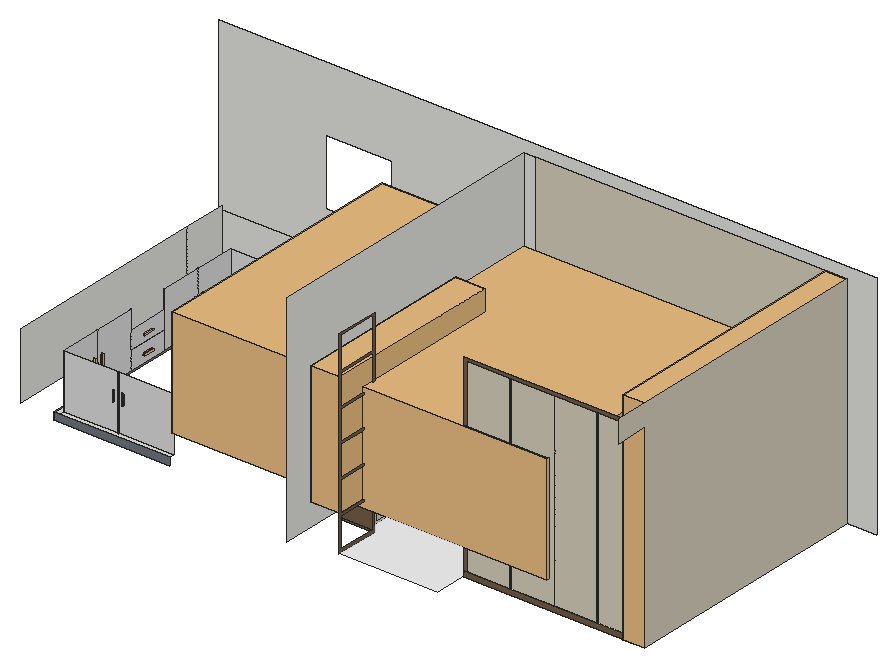
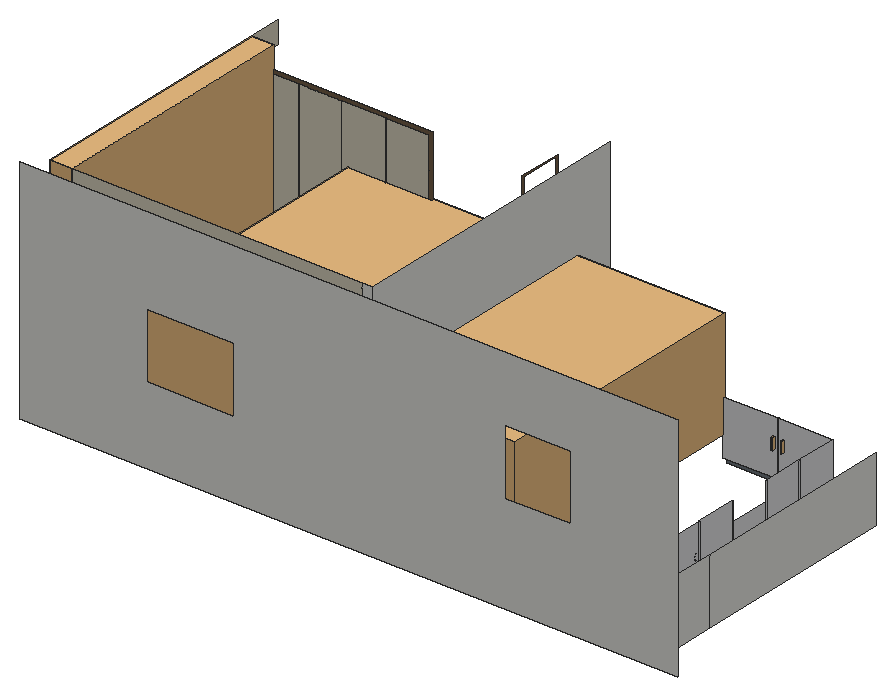
# SketchUp Ruby script. Lengths in inches.
U = 1.inch
M = Sketchup.active_model
def pt(a) = Geom::Point3d.new(a.map { |v| v * U })
def face(e, loops, mat)
  f = e.add_face(loops[0].map { |a| pt(a) })
  loops[1..].each { |l| e.add_face(l.map { |a| pt(a) }).erase! }
  f.material = f.back_material = mat if mat
  f
end
# faces: each face lists its corners as indices into pts; further lists are holes
def faces(e, pts, list, mat = nil) = list.each { |f| face(e, (f[0].is_a?(Array) ? f : [f]).map { |l| l.map { |i| pts[i] } }, mat) }
# xy, xz, yz: faces in a plane at the given z, y or x. An outline is a flat list of corners, or four numbers for a rectangle; further outlines are holes
def ring(l) = l.size == 4 ? [[l[0], l[1]], [l[2], l[1]], [l[2], l[3]], [l[0], l[3]]] : l.each_slice(2).to_a
def flat(e, list, mat, &to3) = list.each { |f| face(e, (f[0].is_a?(Array) ? f : [f]).map { |l| ring(l).map { |u, v| to3.(u, v) } }, mat) }
def xy(e, z, list, mat = nil) = flat(e, list, mat) { |x, y| [x, y, z] }
def xz(e, y, list, mat = nil) = flat(e, list, mat) { |x, z| [x, y, z] }
def yz(e, x, list, mat = nil) = flat(e, list, mat) { |y, z| [x, y, z] }
def lines(e, pts, list) = list.each { |a, b| e.add_line(pt(pts[a]), pt(pts[b])) }
# prism: a flat outline (further loops are holes) pulled along v
def prism(e, loops, v, mat = nil)
  f = face(e, loops, mat); d = Geom::Vector3d.new(v.map { |x| x * U })
  f.pushpull(f.normal.samedirection?(d) ? d.length : -d.length)
end
def box(e, o, s, mat = nil) = prism(e, [[o, [o[0] + s[0], o[1], o[2]], [o[0] + s[0], o[1] + s[1], o[2]], [o[0], o[1] + s[1], o[2]]]], [0, 0, s[2]], mat)
def at(x, y, z, deg = 0) = Geom::Transformation.translation(pt([x, y, z])) * Geom::Transformation.rotation(ORIGIN, Z_AXIS, deg.degrees)
def axes(o, x, y, z) = Geom::Transformation.new([*x, 0, *y, 0, *z, 0, *pt(o).to_a, 1])
def part(name) = M.definitions.add(name)
# library, detail: a bought-in or finely detailed component or shape, given as its bounding box
def library(name, o, s) = part(name).tap { |d| box(d.entities, o, s) }
def detail(e, o, s) = box(e.add_group.entities, o, s)
def put(e, d, t, mat = nil) = e.add_instance(d, t).tap { |i| i.material = mat if mat }
def group(e, t, mat = nil) = e.add_group.tap { |g| g.transformation = t; g.material = mat if mat }.entities
root = M.entities
M.materials.add("1442 AP K091 Frozen Zanskar-N").color = [220, 220, 221]
M.materials.add("1446 AP 8255 STONE PATH").color = [111, 118, 125]
M.materials.add("1689 AP 8482 GREY BUCK").color = [214, 207, 188]
M.materials.add("Tiles Marble White 03 180cm").color = [241, 241, 241]
M.materials["Tiles Marble White 03 180cm"].alpha = 0.94
M.materials.add("Wood Pecan 33-21 150cm").color = [115, 94, 72]
M.materials.add("Wood Walnut 33-38 100cm").color = [48, 31, 12]
M.materials.add("[Mirror 02]").color = [229, 229, 229]
c1 = library("1-POIGNEE CLC2\#1",[-3.03,-0.375,0],[6.06,0.75,1.42])
c2 = library("Shelf decor",[-441.39,577.41,19.36],[99.21,15.9,66.49])
c3 = library("Bedroom+2",[62.69,238.74,0],[145.67,12.71,106.3])
c4 = library("bedroom+kids",[0,0,0],[181.29,144,88.22])
c5 = library("Bedroom+2\#1",[86.24,153.99,0],[98.16,93.56,34.18])
c6 = library("tu+lanh+_+Samsung+Inverter+380+lít+RT38K5982BS.SV",[62.65,2.01,-1.24],[26.58,26.5,71.52])
c7 = library("1-POIGNEE CLC2\#2",[-3.03,-0.375,0],[6.06,0.75,1.42])
xy(root,0,[[134,495,136,531],[172,495,174,531],[9,507,9,531,134,531,134,510,30,510,30,507]])
xy(root,0,[[198,375,252,375,252,392.7,351,392.7,351,531,180,531,180,399,198,399]],"Tiles Marble White 03 180cm")
xy(root,3,[[252,392.7,254,393],[254,392.7,277.45,393],[277.75,392.7,324.95,393],[325.25,392.7,349,393],[349,392.7,351,393]],"1689 AP 8482 GREY BUCK")
xy(root,4,[[30,390,30,507,33,507,33,484.5,32.7,484.5,32.7,484.2,33,484.2,33,461.7,32.7,461.7,32.7,461.4,33,461.4,33,438.9,32.7,438.9,32.7,438.6,33,438.6,33,416.1,32.7,416.1,32.7,415.8,33,415.8,33,390],[33,390,33,393,62.7,393,62.7,392.7,63,392.7,63,393,93,393,93,390],[30,507,30,510,134,510,134,507,100.63,507,100.63,507.3,100.33,507.3,100.33,507,66.97,507,66.97,507.3,66.67,507.3,66.67,507]])
xy(root,4,[[180,399,198,495]],"1689 AP 8482 GREY BUCK")
xy(root,5,[[197.7,431.33,198,431.63],[197.7,462.67,198,462.97]],"1689 AP 8482 GREY BUCK")
xy(root,13.7,[[32.7,438.9,33,461.4],[66.97,507,100.33,507.3]],"1442 AP K091 Frozen Zanskar-N")
xy(root,14,[[32.7,438.9,32.9,461.4],[32.9,438.9,33,461.4],[66.97,507,100.33,507.3]],"1442 AP K091 Frozen Zanskar-N")
xy(root,21,[[197.7,431.33,198,431.63],[197.7,462.67,198,462.97]],"1689 AP 8482 GREY BUCK")
xz(root,390,[[30,0,93,4]],"1446 AP 8255 STONE PATH")
xz(root,392.7,[[62.7,4,63,34]],"1442 AP K091 Frozen Zanskar-N")
xz(root,392.7,[[277.45,3,277.75,106],[324.95,3,325.25,106]],"1689 AP 8482 GREY BUCK")
xz(root,392.7,[[252,0,351,3]],"Wood Pecan 33-21 150cm")
xz(root,393,[[33,4,62.7,34],[63,4,93,34]],"1442 AP K091 Frozen Zanskar-N")
xz(root,393,[[254,3,277.45,106],[277.75,3,301.5,106],[301.5,3,324.95,106],[325.25,3,349,106]],"1689 AP 8482 GREY BUCK")
xz(root,393,[[252,3,252,108,351,108,351,3,349,3,349,106,254,106,254,3]],"Wood Pecan 33-21 150cm")
xz(root,398,[[180,2,198,18.5],[180,19.5,198,22]],"Wood Pecan 33-21 150cm")
xz(root,399,[[180,4,198,22]])
xz(root,399,[[180,0,198,4]],"Wood Pecan 33-21 150cm")
xz(root,415.8,[[32.7,4,33,34]],"1442 AP K091 Frozen Zanskar-N")
xz(root,416.1,[[32.7,4,33,34]],"1442 AP K091 Frozen Zanskar-N")
xz(root,431.33,[[197.7,5,198,21]],"1689 AP 8482 GREY BUCK")
xz(root,431.63,[[197.7,5,198,21]],"1689 AP 8482 GREY BUCK")
xz(root,438.6,[[32.7,4,33,34]],"1442 AP K091 Frozen Zanskar-N")
xz(root,438.9,[[32.7,4,33,13.7],[32.7,14,33,23.7]],"1442 AP K091 Frozen Zanskar-N")
xz(root,461.4,[[32.7,4,33,13.7],[32.7,14,33,23.7]],"1442 AP K091 Frozen Zanskar-N")
xz(root,461.7,[[32.7,4,33,34]])
xz(root,462.67,[[197.7,5,198,21]],"1689 AP 8482 GREY BUCK")
xz(root,462.97,[[197.7,5,198,21]],"1689 AP 8482 GREY BUCK")
xz(root,484.2,[[32.7,4,33,34]],"1442 AP K091 Frozen Zanskar-N")
xz(root,484.5,[[32.7,4,33,34]],"1442 AP K091 Frozen Zanskar-N")
xz(root,495,[[180,4,198,22]])
xz(root,495,[[134,0,136,0,136,70,172,70,172,0,174,0,174,72,134,72]],"Wood Walnut 33-38 100cm")
xz(root,507,[[33,4,66.67,34],[66.97,4,100.33,13.7],[100.63,4,134,34],[66.97,14,100.33,23.7]],"1442 AP K091 Frozen Zanskar-N")
xz(root,507.3,[[66.67,4,66.97,34],[100.33,4,100.63,34],[66.97,13.7,100.33,14]],"1442 AP K091 Frozen Zanskar-N")
xz(root,510,[[30,0,134,4]],"1446 AP 8255 STONE PATH")
xz(root,531,[[9,0,134,4],[134,0,134,72,174,72,174,0,172,0,172,70,136,70,136,0],[174,0,180,120],[9,4,134,34]])
xz(root,531,[[136,0,172,70]],"1442 AP K091 Frozen Zanskar-N")
xz(root,531,[[[180,0,351,0,351,120,180,120,180,30,198,30,198,22,180,22],[243,36,291,72]]],"1689 AP 8482 GREY BUCK")
xz(root,540,[[[0,-6,360,120],[243,36,291,72],[58.6875,48,94.6875,84]]])
yz(root,9,[[393,0,507,36],[507,0,531,36]])
yz(root,30,[[390,0,510,4]],"1446 AP 8255 STONE PATH")
yz(root,32.7,[[415.8,4,416.1,34],[438.6,4,438.9,34],[461.4,4,461.7,34],[484.2,4,484.5,34],[438.9,13.7,461.4,14]],"1442 AP K091 Frozen Zanskar-N")
yz(root,33,[[393,4,415.8,34],[416.1,4,438.6,34],[438.9,4,461.4,13.7],[461.7,4,484.2,34],[484.5,4,507,34],
  [438.9,14,461.4,23.7]],"1442 AP K091 Frozen Zanskar-N")
yz(root,62.7,[[392.7,4,393,34]],"1442 AP K091 Frozen Zanskar-N")
yz(root,63,[[392.7,4,393,34]],"1442 AP K091 Frozen Zanskar-N")
yz(root,66.67,[[507,4,507.3,34]],"1442 AP K091 Frozen Zanskar-N")
yz(root,66.97,[[507,4,507.3,13.7],[507,14,507.3,23.7]])
yz(root,100.33,[[507,4,507.3,13.7]])
yz(root,100.33,[[507,14,507.3,23.7]],"1442 AP K091 Frozen Zanskar-N")
yz(root,100.63,[[507,4,507.3,34]],"1442 AP K091 Frozen Zanskar-N")
yz(root,134,[[510,0,531,4],[507,4,531,34]])
yz(root,134,[[495,0,495,36,505,36,505,34,507,34,507,4,510,4,510,0]],"Wood Walnut 33-38 100cm")
yz(root,136,[[495,0,531,70]],"Wood Walnut 33-38 100cm")
yz(root,172,[[495,0,531,70]],"Wood Walnut 33-38 100cm")
yz(root,174,[[369,0,369,120,531,120,531,72,495,72,495,0]])
yz(root,174,[[495,0,510,72],[510,0,531,72]],"Wood Walnut 33-38 100cm")
yz(root,180,[[399,4,495,22]])
yz(root,180,[[399,0,531,0,531,12,529.76,12.05,528.52,12.13,527.29,12.26,526.06,12.4375,524.83,12.65,523.62,12.91,522.42,13.21,521.22,13.55,520.04,13.93,518.875,14.35,517.72,14.82,516.59,15.32,515.47,15.86,514.37,16.44,513.29,17.05,512.24,17.7,511.2,18.39,510.19,19.12,509.21,19.875,508.26,20.67,507.33,21.49,506.79,22,495,22,495,4,399,4]],"Wood Pecan 33-21 150cm")
yz(root,180,[[531,12,531,22,506.79,22,507.33,21.49,508.26,20.67,509.21,19.875,510.19,19.12,511.2,18.39,512.24,17.7,513.29,17.05,514.37,16.44,515.47,15.86,516.59,15.32,517.72,14.82,518.875,14.35,520.04,13.93,521.22,13.55,522.42,13.21,523.62,12.91,524.83,12.65,526.06,12.4375,527.29,12.26,528.52,12.13,529.76,12.05]],"[Mirror 02]")
yz(root,197.7,[[431.33,5,431.63,21],[462.67,5,462.97,21]],"1689 AP 8482 GREY BUCK")
yz(root,198,[[[399,4,495,22],[400,5,494,21]],[400,5,431.33,21],[431.63,5,462.67,21],[462.97,5,494,21]],"1689 AP 8482 GREY BUCK")
yz(root,198,[[[375,0,399,108],[376,89.5,398,107],[376,72,398,88.5],[376,37,398,53.5],[376,54.5,398,71],[376,2,398,18.5],[376,19.5,398,36]]],"Wood Pecan 33-21 150cm")
yz(root,277.45,[[392.7,3,393,5.5],[392.7,5.5,393,106]],"1689 AP 8482 GREY BUCK")
yz(root,277.75,[[392.7,3,393,5.5],[392.7,5.5,393,106]],"1689 AP 8482 GREY BUCK")
yz(root,324.95,[[392.7,3,393,5.5],[392.7,5.5,393,106]],"1689 AP 8482 GREY BUCK")
yz(root,325.25,[[392.7,3,393,5.5],[392.7,5.5,393,106]],"1689 AP 8482 GREY BUCK")
yz(root,351,[[392.7,0,392.7,3,393,3,393,108,375,108,375,120,531,120,531,0]],"1689 AP 8482 GREY BUCK")
put(root,c1,axes([65.07,393,21.2],[0,0,1],[1,0,0],[0,1,0]))
put(root,c1,axes([59.95,393,21.2],[0,0,1],[1,0,0],[0,1,0]))
put(root,c1,axes([33,413.12,18.57],[0,0,1],[0,-1,0],[1,0,0]))
put(root,c1,axes([33,418.24,18.57],[0,0,1],[0,-1,0],[1,0,0]))
put(root,c2,at(774.45,817.68,0,90))
put(root,c1,axes([33,449.67,8.67],[0,1,0],[0,0,1],[1,0,0]))
put(root,c1,axes([33,449.67,18.67],[0,1,0],[0,0,1],[1,0,0]))
put(root,c3,axes([119.14,590.54,0],[0,-0.94974,0],[0.92208,0,0],[0,0,1.12889]))
put(root,c4,axes([92.81,391.68,15.3],[1.1336,0,0],[0,1,0],[0,0,0.67]))
put(root,c5,at(100.8125,599.11,-0.84,-90))
put(root,c1,axes([33,481.82,18.57],[0,0,1],[0,-1,0],[1,0,0]))
put(root,c1,axes([33,486.94,18.57],[0,0,1],[0,-1,0],[1,0,0]))
put(root,c6,at(78,490.78,0))
put(root,c7,axes([83.73,507,9.15],[1,0,0],[0,0,1],[0,-1,0]))
put(root,c7,axes([83.73,507,19.15],[1,0,0],[0,0,1],[0,-1,0]))
